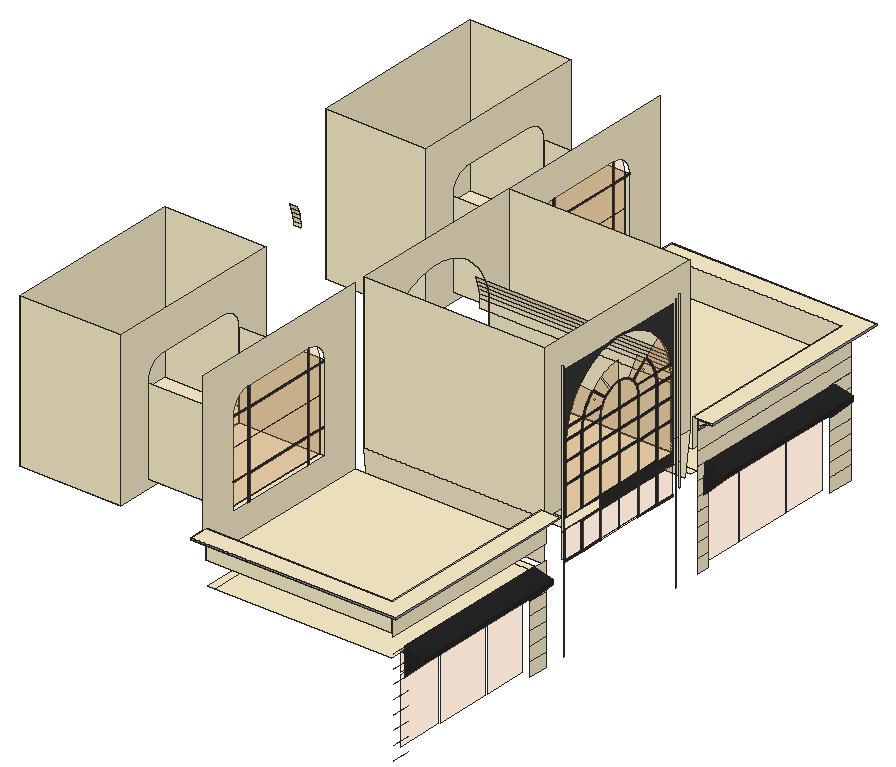
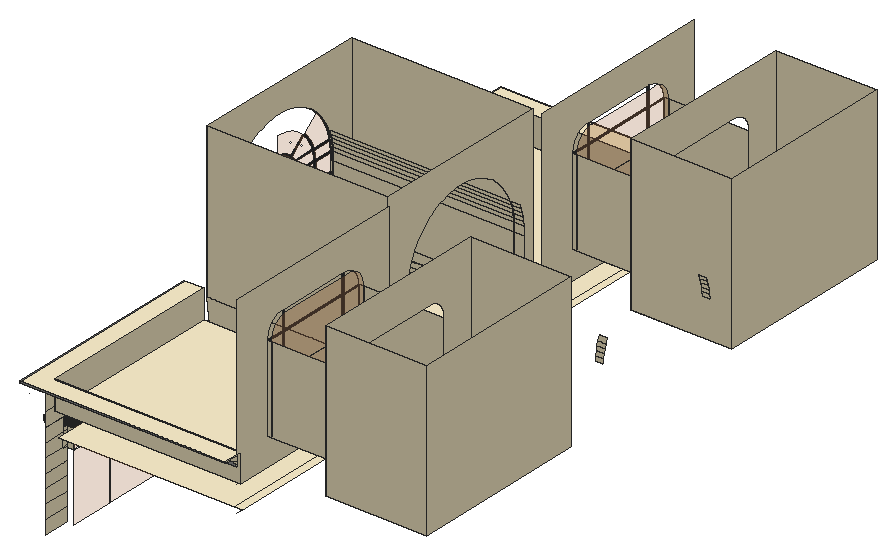
# SketchUp Ruby script. Lengths in inches.
U = 1.inch
M = Sketchup.active_model
def pt(a) = Geom::Point3d.new(a.map { |v| v * U })
def face(e, loops, mat)
  f = e.add_face(loops[0].map { |a| pt(a) })
  loops[1..].each { |l| e.add_face(l.map { |a| pt(a) }).erase! }
  f.material = f.back_material = mat if mat
  f
end
# faces: each face lists its corners as indices into pts; further lists are holes
def faces(e, pts, list, mat = nil) = list.each { |f| face(e, (f[0].is_a?(Array) ? f : [f]).map { |l| l.map { |i| pts[i] } }, mat) }
# xy, xz, yz: faces in a plane at the given z, y or x. An outline is a flat list of corners, or four numbers for a rectangle; further outlines are holes
def ring(l) = l.size == 4 ? [[l[0], l[1]], [l[2], l[1]], [l[2], l[3]], [l[0], l[3]]] : l.each_slice(2).to_a
def flat(e, list, mat, &to3) = list.each { |f| face(e, (f[0].is_a?(Array) ? f : [f]).map { |l| ring(l).map { |u, v| to3.(u, v) } }, mat) }
def xy(e, z, list, mat = nil) = flat(e, list, mat) { |x, y| [x, y, z] }
def xz(e, y, list, mat = nil) = flat(e, list, mat) { |x, z| [x, y, z] }
def yz(e, x, list, mat = nil) = flat(e, list, mat) { |y, z| [x, y, z] }
def lines(e, pts, list) = list.each { |a, b| e.add_line(pt(pts[a]), pt(pts[b])) }
# prism: a flat outline (further loops are holes) pulled along v
def prism(e, loops, v, mat = nil)
  f = face(e, loops, mat); d = Geom::Vector3d.new(v.map { |x| x * U })
  f.pushpull(f.normal.samedirection?(d) ? d.length : -d.length)
end
def box(e, o, s, mat = nil) = prism(e, [[o, [o[0] + s[0], o[1], o[2]], [o[0] + s[0], o[1] + s[1], o[2]], [o[0], o[1] + s[1], o[2]]]], [0, 0, s[2]], mat)
def at(x, y, z, deg = 0) = Geom::Transformation.translation(pt([x, y, z])) * Geom::Transformation.rotation(ORIGIN, Z_AXIS, deg.degrees)
def axes(o, x, y, z) = Geom::Transformation.new([*x, 0, *y, 0, *z, 0, *pt(o).to_a, 1])
def part(name) = M.definitions.add(name)
# library, detail: a bought-in or finely detailed component or shape, given as its bounding box
def library(name, o, s) = part(name).tap { |d| box(d.entities, o, s) }
def detail(e, o, s) = box(e.add_group.entities, o, s)
def put(e, d, t, mat = nil) = e.add_instance(d, t).tap { |i| i.material = mat if mat }
def group(e, t, mat = nil) = e.add_group.tap { |g| g.transformation = t; g.material = mat if mat }.entities
root = M.entities
M.materials.add("Circles_Solid_Black_1K").color = [55, 55, 55]
M.materials.add("D01_Frost_White").color = [255, 242, 206]
M.materials.add("Glass_Safety_01").color = [244, 153, 81]
M.materials["Glass_Safety_01"].alpha = 0.25
M.materials.add("Roofing_02_1K").color = [97, 118, 74]
M.materials.add("ThomThom - Buttons1").color = [48, 49, 53]
M.materials.add("ThomThom - Buttons2").color = [40, 40, 43]
M.materials.add("ThomThom - Hat1").color = [48, 46, 44]
M.materials.add("ThomThom - Hat2").color = [38, 38, 38]
M.materials.add("ThomThom - Waistcoat1").color = [155, 155, 155]
xy(root,42,[[373.34,366.01,374.09,366.03,374.84,366.09,375.59,366.2,376.33,366.35,377.05,366.55,377.77,366.8,378.46,367.09,379.14,367.42,379.79,367.79,380.42,368.21,381.02,368.66,381.59,369.15,382.13,369.68,382.64,370.24,383.1,370.83,383.54,371.44,383.93,372.09,384.28,372.75,384.59,373.44,384.85,374.14,385.07,374.87,385.25,375.6,385.37,376.34,385.45,377.09,385.49,377.84,385.47,378.59,385.41,379.34,385.3,380.09,385.15,380.83,384.95,381.55,384.7,382.27,384.41,382.96,384.08,383.64,383.71,384.29,383.29,384.92,382.84,385.52,382.35,386.09,381.82,386.63,381.26,387.14,380.67,387.6,380.06,388.04,379.41,388.43,378.75,388.78,378.06,389.09,377.36,389.35,376.63,389.57,375.9,389.75,375.16,389.87,374.41,389.95,373.66,389.99,372.91,389.97,372.16,389.91,371.41,389.8,370.67,389.65,369.95,389.45,369.23,389.2,368.54,388.91,367.86,388.58,367.21,388.21,366.58,387.79,365.98,387.34,365.41,386.85,364.87,386.32,364.36,385.76,363.9,385.17,363.46,384.56,363.07,383.91,362.72,383.25,362.41,382.56,362.15,381.86,361.93,381.13,361.75,380.4,361.63,379.66,361.55,378.91,361.51,378.16,361.53,377.41,361.59,376.66,361.7,375.91,361.85,375.17,362.05,374.45,362.3,373.73,362.59,373.04,362.92,372.36,363.29,371.71,363.71,371.08,364.16,370.48,364.65,369.91,365.18,369.37,365.74,368.86,366.33,368.4,366.94,367.96,367.59,367.57,368.25,367.22,368.94,366.91,369.64,366.65,370.37,366.43,371.1,366.25,371.84,366.13,372.59,366.05]],"D01_Frost_White")
xy(root,144,[[252,27,252,258,483,258,483,249,261,249,261,27],[261,27,483,249],[252,498,252,729,261,729,261,507,483,507,483,498],[261,507,483,729],[492,507,516,513],
  [492,705,516,711]],"D01_Frost_White")
xy(root,144,[[483,42,516,234],[483,513,516,705]],"ThomThom - Hat2")
xy(root,174,[[252,24,486,258],[258,294,489,462],[252,498,486,732]],"D01_Frost_White")
xy(root,186,[[258,294,489,462]],"D01_Frost_White")
xy(root,198,[[18,24,144.65,252],[18,504,144.65,732]],"D01_Frost_White")
xy(root,208,[[252,0,252,6,504,6,504,258,510,258,510,0],[252,6,492,18],[492,6,504,258],[492,498,504,738],[504,498,510,738],
  [252,738,504,750],[504,738,510,756],[252,750,504,756]],"D01_Frost_White")
xy(root,210,[[252,0,510,0,510,258,486,258,486,24,252,24],[144.65,66,246,210],[246,66,252,210],[486,498,510,498,510,756,252,756,252,732,486,732],[144.65,546,246,690],
  [246,546,252,690]],"D01_Frost_White")
xz(root,0,[[252,208,510,210]],"ThomThom - Waistcoat1")
xz(root,18,[[252,196,492,202],[252,202,492,208]],"D01_Frost_White")
xz(root,24,[[252,174,486,210],[18,198,144.65,390]],"D01_Frost_White")
xz(root,36,[[492,120,516,144,516,150,492,156]],"ThomThom - Hat2")
xz(root,42,[[492,120,492,144,516,144]],"Roofing_02_1K")
xz(root,66,[[144.65,210,246,318],[246,210,252,318]],"D01_Frost_White")
xz(root,210,[[144.65,210,246,318],[246,210,252,318]],"D01_Frost_White")
xz(root,234,[[492,120,516,144,492,144]],"ThomThom - Hat2")
xz(root,240,[[492,120,492,156,516,150,516,144]],"Roofing_02_1K")
xz(root,252,[[18,198,144.65,390]],"D01_Frost_White")
xz(root,258,[[492,196,498,205,492,202],[492,202,504,208,492,208],[498,205,510,208,504,208]],"D01_Frost_White")
xz(root,264,[[258,198,486,390]],"D01_Frost_White")
xz(root,286,[[490,144,491,174],[490,174,491,362]],"D01_Frost_White")
xz(root,290,[[489,32,490,144],[489,144,490,174],[489,174,490,358]],"D01_Frost_White")
xz(root,294,[[246,174,258,198],[258,186,258,198,486,198,486,264,489,264,489,186],[246,198,258,264],[258,198,486,264],[246,264,258,275.43],
  [258,264,486,275.43],[486,264,489,275.43]],"D01_Frost_White")
xz(root,462,[[258,174,486,186],[486,174,489,186],[258,186,486,264],[486,186,489,264],[246,264,258,275.43],
  [258,264,486,275.43],[486,264,489,275.43]],"D01_Frost_White")
xz(root,466,[[489,32,490,144],[489,144,490,174],[489,174,490,358]],"D01_Frost_White")
xz(root,470,[[490,144,491,174],[490,174,491,362]],"D01_Frost_White")
xz(root,492,[[258,198,486,390]],"D01_Frost_White")
xz(root,498,[[492,196,492,202,498,205],[492,202,492,208,504,208],[498,205,504,208,510,208]],"D01_Frost_White")
xz(root,504,[[18,198,144.65,390]],"D01_Frost_White")
xz(root,507,[[492,120,516,144,492,144],[492,144,516,144,516,150,492,156]],"ThomThom - Hat2")
xz(root,513,[[483,120,492,144]],"D01_Frost_White")
xz(root,513,[[492,120,492,144,516,144]],"ThomThom - Hat2")
xz(root,546,[[144.65,210,246,318],[246,210,252,318]],"D01_Frost_White")
xz(root,690,[[144.65,210,246,318],[246,210,252,318]],"D01_Frost_White")
xz(root,705,[[483,120,492,144]],"D01_Frost_White")
xz(root,705,[[492,120,516,144,492,144]],"ThomThom - Hat2")
xz(root,711,[[492,120,492,144,516,144],[492,144,492,156,516,150,516,144]],"ThomThom - Hat2")
xz(root,732,[[252,174,486,210],[18,198,144.65,390]],"D01_Frost_White")
xz(root,738,[[252,196,492,202],[252,202,492,208]],"D01_Frost_White")
xz(root,756,[[252,208,510,210]],"ThomThom - Waistcoat1")
yz(root,18,[[24,198,252,390],[504,198,732,390]],"D01_Frost_White")
yz(root,144.65,[[[24,198,252,390],[66,210,210,210,210,319.16,209.99,319.52,209.95,320.28,209.89,321.03,209.8,321.79,209.68,322.54,209.54,323.29,209.38,324.03,209.19,324.77,208.98,325.5,208.75,326.22,208.49,326.93,208.21,327.64,207.9,328.33,207.58,329.02,207.23,329.7,206.86,330.36,206.47,331.01,206.05,331.65,205.62,332.27,205.17,332.88,204.69,333.48,204.2,334.06,203.69,334.62,203.16,335.16,202.62,335.69,202.06,336.2,201.48,336.69,200.88,337.17,200.27,337.62,199.65,338.05,199.01,338.47,198.36,338.86,197.7,339.23,197.02,339.58,196.33,339.9,195.64,340.21,194.93,340.49,194.22,340.75,193.5,340.98,192.77,341.19,192.03,341.38,191.29,341.54,190.54,341.68,189.79,341.8,189.03,341.89,188.28,341.95,187.52,341.99,187.16,342,88.1,342,87.71,341.98,86.95,341.93,86.19,341.85,85.4375,341.74,84.68,341.61,83.9375,341.46,83.2,341.28,82.46,341.07,81.73,340.84,81.01,340.59,80.3,340.3125,79.6,340.01,78.91,339.6875,78.23,339.34,77.56,338.97,76.9,338.58,76.26,338.17,75.63,337.74,75.02,337.29,74.42,336.8125,73.84,336.32,73.27,335.81,72.72,335.28,72.19,334.73,71.68,334.16,71.1875,333.58,70.71,332.98,70.26,332.37,69.83,331.74,69.42,331.1,69.03,330.44,68.66,329.77,68.3125,329.09,67.99,328.4,67.6875,327.7,67.41,326.99,67.16,326.27,66.93,325.54,66.72,324.8,66.54,324.0625,66.39,323.32,66.26,322.5625,66.15,321.81,66.07,321.05,66.02,320.29,66,319.9]],[[504,198,732,390],[546,210,690,210,690,319.87,689.98,320.29,689.93,321.05,689.85,321.81,689.74,322.5625,689.61,323.31,689.45,324.0625,689.27,324.8,689.07,325.54,688.84,326.27,688.58,326.98,688.31,327.7,688.01,328.4,687.68,329.09,687.34,329.77,686.97,330.4375,686.58,331.09,686.17,331.73,685.73,332.36,685.28,332.98,684.81,333.57,684.3125,334.16,683.8,334.72,683.27,335.27,682.72,335.8,682.16,336.3125,681.57,336.81,680.98,337.28,680.36,337.73,679.73,338.17,679.09,338.58,678.4375,338.97,677.77,339.34,677.09,339.68,676.4,340.01,675.7,340.31,674.98,340.58,674.27,340.84,673.54,341.07,672.8,341.27,672.0625,341.45,671.31,341.61,670.5625,341.74,669.81,341.85,669.05,341.93,668.29,341.98,667.87,342,567.32,342,566.93,341.98,566.17,341.91,565.41,341.8125,564.65,341.6875,563.9,341.54,563.15,341.37,562.41,341.17,561.68,340.95,560.95,340.7,560.23,340.43,559.53,340.13,558.83,339.8125,558.14,339.47,557.47,339.1,556.81,338.71,556.16,338.3,555.53,337.87,554.91,337.42,554.31,336.94,553.72,336.45,553.15,335.93,552.6,335.4,552.07,334.85,551.55,334.28,551.06,333.69,550.58,333.09,550.13,332.47,549.7,331.84,549.29,331.19,548.9,330.53,548.53,329.86,548.1875,329.17,547.87,328.47,547.57,327.77,547.3,327.05,547.05,326.32,546.83,325.59,546.63,324.85,546.46,324.1,546.3125,323.35,546.1875,322.59,546.09,321.83,546.02,321.07,546,320.68]]],"D01_Frost_White")
yz(root,246,[[66,210,210,275.23],[546,210,690,275.23],[66,275.23,66,319.9,66.02,320.29,66.07,321.05,66.15,321.81,66.26,322.5625,66.39,323.32,66.54,324.0625,66.72,324.8,66.93,325.54,67.16,326.27,67.41,326.99,67.6875,327.7,67.99,328.4,68.3125,329.09,68.66,329.77,69.03,330.44,69.42,331.1,69.83,331.74,70.26,332.37,70.71,332.98,71.1875,333.58,71.68,334.16,72.19,334.73,72.72,335.28,73.27,335.81,73.84,336.32,74.42,336.8125,75.02,337.29,75.63,337.74,76.26,338.17,76.9,338.58,77.56,338.97,78.23,339.34,78.91,339.6875,79.6,340.01,80.3,340.3125,81.01,340.59,81.73,340.84,82.46,341.07,83.2,341.28,83.9375,341.46,84.68,341.61,85.4375,341.74,86.19,341.85,86.95,341.93,87.71,341.98,88.1,342,187.16,342,187.52,341.99,188.28,341.95,189.03,341.89,189.79,341.8,190.54,341.68,191.29,341.54,192.03,341.38,192.77,341.19,193.5,340.98,194.22,340.75,194.93,340.49,195.64,340.21,196.33,339.9,197.02,339.58,197.7,339.23,198.36,338.86,199.01,338.47,199.65,338.05,200.27,337.62,200.88,337.17,201.48,336.69,202.06,336.2,202.62,335.69,203.16,335.16,203.69,334.62,204.2,334.06,204.69,333.48,205.17,332.88,205.62,332.27,206.05,331.65,206.47,331.01,206.86,330.36,207.23,329.7,207.58,329.02,207.9,328.33,208.21,327.64,208.49,326.93,208.75,326.22,208.98,325.5,209.19,324.77,209.38,324.03,209.54,323.29,209.68,322.54,209.8,321.79,209.89,321.03,209.95,320.28,209.99,319.52,210,319.16,210,275.23],[546,275.23,546,320.68,546.02,321.07,546.09,321.83,546.1875,322.59,546.3125,323.35,546.46,324.1,546.63,324.85,546.83,325.59,547.05,326.32,547.3,327.05,547.57,327.77,547.87,328.47,548.1875,329.17,548.53,329.86,548.9,330.53,549.29,331.19,549.7,331.84,550.13,332.47,550.58,333.09,551.06,333.69,551.55,334.28,552.07,334.85,552.6,335.4,553.15,335.93,553.72,336.45,554.31,336.94,554.91,337.42,555.53,337.87,556.16,338.3,556.81,338.71,557.47,339.1,558.14,339.47,558.83,339.8125,559.53,340.13,560.23,340.43,560.95,340.7,561.68,340.95,562.41,341.17,563.15,341.37,563.9,341.54,564.65,341.6875,565.41,341.8125,566.17,341.91,566.93,341.98,567.32,342,667.87,342,668.29,341.98,669.05,341.93,669.81,341.85,670.5625,341.74,671.31,341.61,672.0625,341.45,672.8,341.27,673.54,341.07,674.27,340.84,674.98,340.58,675.7,340.31,676.4,340.01,677.09,339.68,677.77,339.34,678.4375,338.97,679.09,338.58,679.73,338.17,680.36,337.73,680.98,337.28,681.57,336.81,682.16,336.3125,682.72,335.8,683.27,335.27,683.8,334.72,684.3125,334.16,684.81,333.57,685.28,332.98,685.73,332.36,686.17,331.73,686.58,331.09,686.97,330.4375,687.34,329.77,687.68,329.09,688.01,328.4,688.31,327.7,688.58,326.98,688.84,326.27,689.07,325.54,689.27,324.8,689.45,324.0625,689.61,323.31,689.74,322.5625,689.85,321.81,689.93,321.05,689.98,320.29,690,319.87,690,275.23]],"Glass_Safety_01")
yz(root,252,[[[24,174,258,174,258,384,18,384,18,210,24,210],[66,210,66,318,65.98,318.76,65.98,319.53,66,319.9,66.02,320.29,66.07,321.05,66.15,321.81,66.26,322.5625,66.39,323.32,66.54,324.0625,66.72,324.8,66.93,325.54,67.16,326.27,67.41,326.99,67.6875,327.7,67.99,328.4,68.3125,329.09,68.66,329.77,69.03,330.44,69.42,331.1,69.83,331.74,70.26,332.37,70.71,332.98,71.1875,333.58,71.68,334.16,72.19,334.73,72.72,335.28,73.27,335.81,73.84,336.32,74.42,336.8125,75.02,337.29,75.63,337.74,76.26,338.17,76.9,338.58,77.56,338.97,78.23,339.34,78.91,339.6875,79.6,340.01,80.3,340.3125,81.01,340.59,81.73,340.84,82.46,341.07,83.2,341.28,83.9375,341.46,84.68,341.61,85.4375,341.74,86.19,341.85,86.95,341.93,87.71,341.98,88.1,342,88.47,342.02,89.24,342.02,90,342,186,342,186.76,342.01,187.16,342,187.52,341.99,188.28,341.95,189.03,341.89,189.79,341.8,190.54,341.68,191.29,341.54,192.03,341.38,192.77,341.19,193.5,340.98,194.22,340.75,194.93,340.49,195.64,340.21,196.33,339.9,197.02,339.58,197.7,339.23,198.36,338.86,199.01,338.47,199.65,338.05,200.27,337.62,200.88,337.17,201.48,336.69,202.06,336.2,202.62,335.69,203.16,335.16,203.69,334.62,204.2,334.06,204.69,333.48,205.17,332.88,205.62,332.27,206.05,331.65,206.47,331.01,206.86,330.36,207.23,329.7,207.58,329.02,207.9,328.33,208.21,327.64,208.49,326.93,208.75,326.22,208.98,325.5,209.19,324.77,209.38,324.03,209.54,323.29,209.68,322.54,209.8,321.79,209.89,321.03,209.95,320.28,209.99,319.52,210,319.16,210.01,318.76,210,318,210,210]],[[498,174,732,174,732,210,738,210,738,384,498,384],[546,210,546,318,545.97,318.77,545.96,319.53,545.98,320.3,546,320.68,546.02,321.07,546.09,321.83,546.1875,322.59,546.3125,323.35,546.46,324.1,546.63,324.85,546.83,325.59,547.05,326.32,547.3,327.05,547.57,327.77,547.87,328.47,548.1875,329.17,548.53,329.86,548.9,330.53,549.29,331.19,549.7,331.84,550.13,332.47,550.58,333.09,551.06,333.69,551.55,334.28,552.07,334.85,552.6,335.4,553.15,335.93,553.72,336.45,554.31,336.94,554.91,337.42,555.53,337.87,556.16,338.3,556.81,338.71,557.47,339.1,558.14,339.47,558.83,339.8125,559.53,340.13,560.23,340.43,560.95,340.7,561.68,340.95,562.41,341.17,563.15,341.37,563.9,341.54,564.65,341.6875,565.41,341.8125,566.17,341.91,566.93,341.98,567.32,342,567.7,342.02,568.47,342.04,569.23,342.03,570,342,666,342,666.76,342.02,667.53,342.01,667.87,342,668.29,341.98,669.05,341.93,669.81,341.85,670.5625,341.74,671.31,341.61,672.0625,341.45,672.8,341.27,673.54,341.07,674.27,340.84,674.98,340.58,675.7,340.31,676.4,340.01,677.09,339.68,677.77,339.34,678.4375,338.97,679.09,338.58,679.73,338.17,680.36,337.73,680.98,337.28,681.57,336.81,682.16,336.3125,682.72,335.8,683.27,335.27,683.8,334.72,684.3125,334.16,684.81,333.57,685.28,332.98,685.73,332.36,686.17,331.73,686.58,331.09,686.97,330.4375,687.34,329.77,687.68,329.09,688.01,328.4,688.31,327.7,688.58,326.98,688.84,326.27,689.07,325.54,689.27,324.8,689.45,324.0625,689.61,323.31,689.74,322.5625,689.85,321.81,689.93,321.05,689.98,320.29,690,319.87,690.01,319.53,690.02,318.76,690,318,690,210]],[18,196,12,205,18,202],[738,196,738,202,744,205],[18,202,6,208,18,208],
  [738,202,738,208,750,208],[12,205,0,208,6,208],[744,205,750,208,756,208],[0,208,18,210],[738,208,756,210]],"D01_Frost_White")
yz(root,252,[[[90,210,92,210,92,242,184,242,184,210,186,210,186,242,210,242,210,244,186,244,186,316,210,316,210,318,186,318,186,342,184,342,184,318,92,318,92,342,90,342,90,318,66,318,66,316,90,316,90,244,66,244,66,242,90,242],[92,244,184,316]],[[570,210,572,210,572,242,664,242,664,210,666,210,666,242,690,242,690,244,666,244,666,316,690,316,690,318,666,318,666,342,664,342,664,318,572,318,572,342,570,342,570,318,546,318,546,316,570,316,570,244,546,244,546,242,570,242],[572,244,664,316]]],"ThomThom - Buttons1")
yz(root,258,[[294,174,462,186],[264,198,294,198,294,275.43,294.49,280.53,295.37,285.98,296.61,291.37,298.2,296.65,300.13,301.83,302.4,306.86,304.99,311.74,307.89,316.43,311.1,320.93,314.59,325.2,318.36,329.24,322.39,333.02,326.65,336.53,331.13,339.75,335.82,342.67,340.6875,345.28,345.71,347.5625,350.88,349.51,356.16,351.12,361.54,352.375,366.99,353.28,372.48,353.82,378,354,383.52,353.82,389.01,353.28,394.46,352.375,399.84,351.12,405.12,349.51,410.29,347.5625,415.3125,345.28,420.18,342.67,424.87,339.75,429.35,336.53,433.61,333.02,437.64,329.24,441.41,325.2,444.9,320.93,448.11,316.43,451.01,311.74,453.6,306.86,455.87,301.83,457.8,296.65,459.39,291.37,460.63,285.98,461.51,280.53,462,275.43,462,198,492,198,492,390,264,390]],"D01_Frost_White")
yz(root,483,[[513,34,573,118],[575,34,647,118],[649,34,705,118],[42,36,102,118],[104,36,176,118],
  [178,36,234,118],[42,120,102,144],[104,120,176,144],[178,120,234,144],[513,120,573,144],
  [575,120,647,144],[649,120,705,144]],"Glass_Safety_01")
yz(root,486,[[24,174,258,210],[498,174,732,210],[264,198,264,390,492,390,492,198,462,198,462,275.43,461.51,280.53,460.63,285.98,459.39,291.37,457.8,296.65,455.87,301.83,453.6,306.86,451.01,311.74,448.11,316.43,444.9,320.93,441.41,325.2,437.64,329.24,433.61,333.02,429.35,336.53,424.87,339.75,420.18,342.67,415.3125,345.28,410.29,347.5625,405.12,349.51,399.84,351.12,394.46,352.375,389.01,353.28,383.52,353.82,378,354,372.48,353.82,366.99,353.28,361.54,352.375,356.16,351.12,350.88,349.51,345.71,347.5625,340.6875,345.28,335.82,342.67,331.13,339.75,326.65,336.53,322.39,333.02,318.36,329.24,314.59,325.2,311.1,320.93,307.89,316.43,304.99,311.74,302.4,306.86,300.13,301.83,298.2,296.65,296.61,291.37,295.37,285.98,294.49,280.53,294,275.43,294,198]],"D01_Frost_White")
yz(root,489,[[294,275.43,294.49,280.53,295.37,285.98,295.42,286.1875,295.88,288.1875,296.61,291.37,298.2,296.65,300.13,301.83,302.4,306.86,304.99,311.74,307.89,316.43,311.1,320.93,314.59,325.2,316.37,327.1,317.4,328.21,318.36,329.24,322.39,333.02,326.65,336.53,331.13,339.75,333.04,340.94,334.65,341.94,335.82,342.67,340.6875,345.28,345.71,347.5625,350.88,349.51,356.16,351.12,361.54,352.375,366.99,353.28,372.48,353.82,377,353.97,377,354,294,354],[462,275.43,462,354,379,354,379,353.97,383.52,353.82,389.01,353.28,394.46,352.375,399.84,351.12,405.12,349.51,410.29,347.5625,415.3125,345.28,420.18,342.67,421.22,342.02,422.83,341.02,424.87,339.75,429.35,336.53,433.61,333.02,437.64,329.24,438.53,328.29,439.55,327.19,441.41,325.2,444.9,320.93,448.11,316.43,451.01,311.74,453.6,306.86,455.87,301.83,457.8,296.65,459.39,291.37,460.12,288.1875,460.58,286.1875,460.63,285.98,461.51,280.53]],"Circles_Solid_Black_1K")
yz(root,489,[[294,264,294,275.43,293.96,275.04,293.8,269.52],[462,264,462.2,269.52,462.0625,274.1875,462,274.1875],[462,274.1875,462.0625,274.1875,462.04,275.04,462,275.43]],"D01_Frost_White")
yz(root,489,[[348.5,136.9,377,138.9],[377,136.9,379,138.9],[379,136.9,407.5,138.9],[294,138.9,318,174],[320,138.9,347.5,172],
  [348.5,138.9,377,172],[377,138.9,379,172],[379,138.9,407.5,172],[408.5,138.9,436,172],[438,138.9,462,174],
  [294,186,318,222.1875],[438,186,462,222.1875],[320,188,347.5,222.1875],[348.5,188,377,222.1875],[379,188,407.5,222.1875],
  [408.5,188,436,222.1875],[294,224.1875,318,248.1875],[320,224.1875,347.5,248.1875],[348.5,224.1875,377,248.1875],[379,224.1875,407.5,248.1875],
  [408.5,224.1875,436,248.1875],[438,224.1875,462,248.1875],[294,250.1875,318,272.1875],[320,250.1875,347.5,272.1875],[348.5,250.1875,377,272.1875],
  [379,250.1875,407.5,272.1875],[408.5,250.1875,436,272.1875],[438,250.1875,462,272.1875],[294,274.1875,318,274.1875,318,274.28,318.3,277.47,318.94,281.37,319.82,285.22,320.11,286.1875,295.42,286.1875,295.37,285.98,294.49,280.53,294,275.43],[320,274.1875,347.5,274.1875,347.56,276.1,347.74,278.01,348.04,279.9,348.46,281.77,348.99,283.61,349.64,285.42,349.98,286.1875,322.2,286.1875,321.75,284.7,320.9,280.98,320.29,277.22],
  [[348.5,274.1875,377,274.1875,377,303.66,376.15,303.63,374.3,303.46,372.47,303.17,370.66,302.76,368.88,302.24,367.14,301.62,365.44,300.88,363.79,300.04,362.19,299.1,360.66,298.05,359.2,296.92,357.81,295.69,356.5,294.38,355.27,292.99,354.13,291.53,353.09,290,352.15,288.4,352.04,288.1875,351.31,286.75,351.07,286.1875,350.57,285.05,349.94,283.3,349.43,281.52,349.02,279.72,348.73,277.89,348.56,276.04],[347.5,188,348.5,222.1875],[347.5,224.1875,348.5,248.1875],[347.5,250.1875,348.5,272.1875]],[379,274.1875,407.5,274.1875,407.44,276.04,407.27,277.89,406.98,279.72,406.57,281.52,406.06,283.3,405.43,285.05,404.93,286.1875,404.69,286.75,403.96,288.1875,403.85,288.4,402.91,290,401.87,291.53,400.73,292.99,399.5,294.38,398.19,295.69,396.8,296.92,395.34,298.05,393.81,299.1,392.21,300.04,390.56,300.88,388.86,301.62,387.12,302.24,385.34,302.76,383.53,303.17,381.7,303.46,379.85,303.63,379,303.66],[408.5,274.1875,436,274.1875,435.71,277.22,435.1,280.98,434.25,284.7,433.8,286.1875,406.02,286.1875,406.36,285.42,407.01,283.61,407.54,281.77,407.96,279.9,408.26,278.01,408.44,276.1],[438,274.1875,462,274.1875,462,275.43,461.51,280.53,460.63,285.98,460.58,286.1875,435.89,286.1875,436.18,285.22,437.06,281.37,437.7,277.47,438,274.28],[295.88,288.1875,320.71,288.1875,320.96,289,322.34,292.69,323.96,296.29,325.81,299.78,327.89,303.13,330.18,306.35,332.68,309.4,334.82,311.7,316.37,327.1,314.59,325.2,311.1,320.93,307.89,316.43,304.99,311.74,302.4,306.86,300.13,301.83,298.2,296.65,296.61,291.37],
  [[322.8,288.1875,350.92,288.1875,351.27,288.88,352.25,290.53,353.32,292.12,354.5,293.63,355.77,295.07,357.12,296.42,358.56,297.6875,360.07,298.86,361.66,299.94,363.31,300.92,365.01,301.79,366.77,302.55,368.57,303.2,370.41,303.73,372.28,304.15,374.18,304.45,376.08,304.63,377,304.66,377,327.95,374.1875,327.86,370.39,327.49,366.625,326.86,362.91,325.99,359.26,324.89,355.6875,323.54,352.21,321.96,350.4,320.99,364.82,301.79,363.12,300.92,348.72,320.08,345.61,318.14,342.51,315.91,339.57,313.49,337.43,311.47,356.25,295.74,355.58,295.07,355.22,294.67,336.36,310.42,334.18,308.09,331.77,305.13,329.55,302.03,327.54,298.78,325.75,295.41,324.1875,291.93,322.85,288.36],[338.87,299.58,338.92,299.66,338.96,299.71]],[[405.08,288.1875,433.2,288.1875,433.15,288.36,431.8125,291.93,430.25,295.41,428.46,298.78,426.45,302.03,424.23,305.13,421.82,308.09,419.56,310.51,400.58,294.67,401.5,293.63,402.68,292.12,403.75,290.53,404.73,288.88],[417.13,299.58,417.04,299.71,417.08,299.66]],[435.29,288.1875,460.12,288.1875,459.39,291.37,457.8,296.65,455.87,301.83,453.6,306.86,451.01,311.74,448.11,316.43,444.9,320.93,441.41,325.2,439.55,327.19,421.1,311.79,423.32,309.4,425.82,306.35,428.11,303.13,430.19,299.78,432.04,296.29,433.66,292.69,435.04,289],[399.56,295.74,418.48,311.56,416.43,313.49,413.49,315.91,410.39,318.14,407.15,320.16,392.69,300.92,394.34,299.94,395.93,298.86,397.44,297.6875,398.88,296.42]],"Glass_Safety_01")
yz(root,489,[[294,136.9,318,138.9],[320,136.9,347.5,138.9],[408.5,136.9,436,138.9],[438,136.9,462,138.9],[355.22,294.67,355.58,295.07,356.25,295.74,337.43,311.47,336.79,310.875,336.36,310.42],
  [400.58,294.67,419.56,310.51,418.48,311.56,399.56,295.74,400.23,295.07]],"ThomThom - Buttons1")
yz(root,489,[[318,136.9,320,138.9],[347.5,136.9,348.5,138.9],[407.5,136.9,408.5,138.9],[436,136.9,438,138.9],[318,138.9,320,138.9,320,172,347.5,172,347.5,174,318,174],
  [347.5,138.9,348.5,172],[407.5,138.9,408.5,172],[436,138.9,438,138.9,438,174,408.5,174,408.5,172,436,172],[347.5,172,348.5,174],[348.5,172,377,174],
  [377,172,379,174],[379,172,407.5,174],[407.5,172,408.5,174],[318,186,347.5,186,347.5,188,320,188,320,222.1875,347.5,222.1875,347.5,224.1875,320,224.1875,320,248.1875,347.5,248.1875,347.5,250.1875,320,250.1875,320,272.1875,347.5,272.1875,347.5,274.1875,320,274.1875,320.29,277.22,320.9,280.98,321.75,284.7,322.2,286.1875,349.98,286.1875,350.4,287.17,350.92,288.1875,322.8,288.1875,322.85,288.36,324.1875,291.93,325.75,295.41,327.54,298.78,329.55,302.03,331.77,305.13,334.18,308.09,336.36,310.42,336.25,310.51,334.82,311.7,332.68,309.4,330.18,306.35,327.89,303.13,325.81,299.78,323.96,296.29,322.34,292.69,320.96,289,320.71,288.1875,295.88,288.1875,295.42,286.1875,320.11,286.1875,319.82,285.22,318.94,281.37,318.3,277.47,318,274.28,318,274.1875,294,274.1875,294,272.1875,318,272.1875,318,250.1875,294,250.1875,294,248.1875,318,248.1875,318,224.1875,294,224.1875,294,222.1875,318,222.1875],[347.5,186,348.5,188],
  [348.5,186,377,188],[377,186,379,188],[379,186,407.5,188],[408.5,186,438,186,438,222.1875,462,222.1875,462,224.1875,438,224.1875,438,248.1875,462,248.1875,462,250.1875,438,250.1875,438,272.1875,462,272.1875,462,274.1875,438,274.1875,438,274.28,437.7,277.47,437.06,281.37,436.18,285.22,435.89,286.1875,460.58,286.1875,460.12,288.1875,435.29,288.1875,435.04,289,433.66,292.69,432.04,296.29,430.19,299.78,428.11,303.13,425.82,306.35,423.32,309.4,421.1,311.79,419.56,310.51,421.82,308.09,424.23,305.13,426.45,302.03,428.46,298.78,430.25,295.41,431.8125,291.93,433.15,288.36,433.2,288.1875,405.08,288.1875,405.6,287.17,406.02,286.1875,433.8,286.1875,434.25,284.7,435.1,280.98,435.71,277.22,436,274.1875,408.5,274.1875,408.5,272.1875,436,272.1875,436,250.1875,408.5,250.1875,408.5,248.1875,436,248.1875,436,224.1875,408.5,224.1875,408.5,222.1875,436,222.1875,436,188,408.5,188],[407.5,186,408.5,188],
  [347.5,188,348.5,222.1875],[377,188,379,188,379,222.1875,407.5,222.1875,407.5,224.1875,379,224.1875,379,248.1875,407.5,248.1875,407.5,250.1875,379,250.1875,379,272.1875,407.5,272.1875,407.5,274.1875,379,274.1875,379,303.66,378,303.6875,377,303.66,377,274.1875,348.5,274.1875,348.5,272.1875,377,272.1875,377,250.1875,348.5,250.1875,348.5,248.1875,377,248.1875,377,224.1875,348.5,224.1875,348.5,222.1875,377,222.1875],[407.5,188,408.5,222.1875],[347.5,222.1875,348.5,224.1875],[407.5,222.1875,408.5,224.1875],
  [347.5,224.1875,348.5,248.1875],[407.5,224.1875,408.5,248.1875],[347.5,248.1875,348.5,250.1875],[407.5,248.1875,408.5,250.1875],[347.5,250.1875,348.5,272.1875],
  [407.5,250.1875,408.5,272.1875],[347.5,272.1875,348.5,274.1875],[407.5,272.1875,408.5,274.1875],[347.5,274.1875,348.5,274.1875,348.56,276.04,348.73,277.89,349.02,279.72,349.43,281.52,349.94,283.3,350.57,285.05,351.07,286.1875,349.98,286.1875,349.64,285.42,348.99,283.61,348.46,281.77,348.04,279.9,347.74,278.01,347.56,276.1],[407.5,274.1875,408.5,274.1875,408.44,276.1,408.26,278.01,407.96,279.9,407.54,281.77,407.01,283.61,406.36,285.42,406.02,286.1875,404.93,286.1875,405.43,285.05,406.06,283.3,406.57,281.52,406.98,279.72,407.27,277.89,407.44,276.04],
  [349.98,286.1875,351.07,286.1875,351.31,286.75,352.04,288.1875,350.92,288.1875,350.4,287.17],[404.93,286.1875,406.02,286.1875,405.6,287.17,405.08,288.1875,403.96,288.1875,404.69,286.75],[350.92,288.1875,352.04,288.1875,352.15,288.4,353.09,290,354.13,291.53,355.27,292.99,356.5,294.38,357.81,295.69,359.2,296.92,360.66,298.05,362.19,299.1,363.79,300.04,365.44,300.88,367.14,301.62,368.88,302.24,370.66,302.76,372.47,303.17,374.3,303.46,376.15,303.63,377,303.66,377,304.66,376.08,304.63,374.18,304.45,372.28,304.15,370.41,303.73,368.57,303.2,366.77,302.55,365.01,301.79,363.31,300.92,361.66,299.94,360.07,298.86,358.56,297.6875,357.12,296.42,355.77,295.07,354.5,293.63,353.32,292.12,352.25,290.53,351.27,288.88],[403.96,288.1875,405.08,288.1875,404.73,288.88,403.75,290.53,402.68,292.12,401.5,293.63,400.58,294.67,399.56,295.74,398.88,296.42,397.44,297.6875,395.93,298.86,394.34,299.94,392.69,300.92,390.99,301.79,389.23,302.55,387.43,303.2,385.59,303.73,383.72,304.15,381.82,304.45,379.92,304.63,379,304.66,379,303.66,379.85,303.63,381.7,303.46,383.53,303.17,385.34,302.76,387.12,302.24,388.86,301.62,390.56,300.88,392.21,300.04,393.81,299.1,395.34,298.05,396.8,296.92,398.19,295.69,399.5,294.38,400.73,292.99,401.87,291.53,402.91,290,403.85,288.4],[400.58,294.67,400.23,295.07,399.56,295.74]],"ThomThom - Buttons2")
yz(root,489,[[347.5,174,348.5,186],[348.5,174,377,186],[377,174,379,186],[379,174,407.5,186],[407.5,174,408.5,186],
  [408.5,174,462,186]],"ThomThom - Hat1")
yz(root,492,[[234,34.38,258,51.57],[498,34.8,513,52.2],[705,34.8,738,52.2],[234,51.57,258,68.76],[498,52.2,513,69.6],
  [705,52.2,738,69.6],[234,68.76,258,85.95],[498,69.6,513,87],[705,69.6,738,87],[234,85.95,258,103.14],
  [498,87,513,104.4],[705,87,738,104.4],[234,103.14,258,103.14,258,120.32,240,120.32,240,120,234,120],[498,104.4,513,104.4,513,120,507,120,507,121.8,498,121.8],[705,104.4,738,104.4,738,121.8,711,121.8,711,120,705,120],
  [36,120,42,144],[234,120,240,120.32],[507,120,513,121.8],[705,120,711,121.8],[234,120.32,240,137.51],
  [240,120.32,258,137.51],[498,121.8,507,139.2],[507,121.8,513,139.2],[705,121.8,711,139.2],[711,121.8,738,139.2],
  [234,137.51,240,144],[240,137.51,258,154.7],[498,139.2,507,139.2,507,156,711,156,711,139.2,738,139.2,738,174,498,174],[507,139.2,513,144],[705,139.2,711,144],
  [18,174,258,196],[498,174,738,196],[18,196,258,202],[498,196,738,202],[18,202,258,208],
  [498,202,738,208]],"D01_Frost_White")
yz(root,510,[[0,208,258,210],[498,208,756,210]],"ThomThom - Waistcoat1")
yz(root,516,[[36,144,240,150],[507,144,711,150]],"ThomThom - Hat2")
p = [[492,42,120],[516,42,144],[516,36,144],[492,36,120],[516,234,144],[492,234,120],
  [492,240,120],[516,240,144],[492,513,120],[516,513,144],[516,507,144],[492,507,120],
  [492,711,120],[516,711,144],[516,705,144],[492,705,120],[261,267,144],[258,264,198],
  [486,264,198],[483,267,144],[483,489,144],[486,492,198],[258,492,198],[261,489,144],
  [492,36,156],[516,36,150],[516,240,150],[492,240,156],[516,711,150],[492,711,156],
  [492,507,156],[516,507,150],[252,12,205],[252,18,196],[492,18,196],[498,12,205],
  [492,258,196],[498,258,205],[492,18,202],[492,738,196],[498,744,205],[498,498,205],
  [492,498,196],[252,738,196],[252,744,205],[492,738,202],[252,18,202],[492,258,202],
  [492,498,202],[252,738,202],[252,0,208],[510,0,208],[510,258,208],[252,6,208],
  [504,6,208],[492,6,208],[504,258,208],[504,498,208],[504,750,208],[504,738,208],
  [510,498,208],[510,756,208],[510,738,208],[252,750,208],[252,756,208],[504,756,208],
  [21,294.49,280.53],[21,294,275.43],[12,294,275.43],[12,294.49,280.53],[258,294.49,280.53],[258,294,275.43],
  [246,294,275.43],[246,294.49,280.53],[486,294.49,280.53],[486,294,275.43],[489,294.49,280.53],[489,294,275.43],
  [21,462,275.43],[21,461.51,280.53],[12,461.51,280.53],[12,462,275.43],[258,462,275.43],[258,461.51,280.53],
  [246,461.51,280.53],[246,462,275.43],[486,462,275.43],[486,461.51,280.53],[489,462,275.43],[489,461.51,280.53],
  [21,295.37,285.98],[12,295.37,285.98],[258,295.37,285.98],[246,295.37,285.98],[486,295.37,285.98],[489,295.37,285.98],
  [21,460.63,285.98],[12,460.63,285.98],[258,460.63,285.98],[246,460.63,285.98],[486,460.63,285.98],[489,460.63,285.98],
  [21,296.61,291.37],[12,296.61,291.37],[258,296.61,291.37],[246,296.61,291.37],[486,296.61,291.37],[489,295.42,286.1875],
  [489,296.61,291.37],[489,295.88,288.1875],[21,459.39,291.37],[12,459.39,291.37],[258,459.39,291.37],[246,459.39,291.37],
  [486,459.39,291.37],[489,460.12,288.1875],[489,459.39,291.37],[489,460.58,286.1875],[21,298.2,296.65],[12,298.2,296.65],
  [258,298.2,296.65],[246,298.2,296.65],[486,298.2,296.65],[489,298.2,296.65],[21,457.8,296.65],[12,457.8,296.65],
  [258,457.8,296.65],[246,457.8,296.65],[486,457.8,296.65],[489,457.8,296.65],[21,300.13,301.83],[12,300.13,301.83],
  [258,300.13,301.83],[246,300.13,301.83],[486,300.13,301.83],[489,300.13,301.83],[21,455.87,301.83],[12,455.87,301.83],
  [258,455.87,301.83],[246,455.87,301.83],[486,455.87,301.83],[489,455.87,301.83],[252,738.1,176.27],[252,738,176.27],
  [492,18,34.51],[492,42,34.51],[492,18,51.77],[492,42,51.77],[492,18,69.03],[492,42,69.03],
  [492,18,86.29],[492,42,86.29],[492,18,103.54],[492,42,103.54],[492,18,120.8],[492,42,120.8],
  [492,18,138.06],[492,42,138.06],[492,18,155.32],[492,42,155.32],[492,178,144],[492,176,144],
  [492,104,144],[492,102,144],[489,463.28,274.1875],[489,462.0625,274.1875],[504,750,196],[504.07,750,196],
  [489,294,174],[491,462,174],[489,295.37,286.1875],[489,460.37,288.1875],[489,295.42,288.1875],[252,729,144],
  [252,738,144],[492,234,154.7],[492,240,154.7],[492,738,156.6],[492,705,156.6],[492,513,156.6],
  [492,498,156.6]]
faces(root,p,[[0,1,2,3],[4,5,6,7],[8,9,10,11],[12,13,14,15],[24,25,26,27],[28,29,30,31]],"ThomThom - Hat2")
faces(root,p,[[16,17,18,19],[20,21,22,23],[34,35,38],[40,39,45],[38,35,32,46],[47,37,35,38],[45,40,41,48],[49,44,40,45],
  [53,32,35,54,55],[54,35,37,56],[57,41,40,58,59],[58,40,44,63],[66,67,68,69],[70,71,72,73],[74,75,71,70],[76,77,75,74],
  [78,79,80,81],[82,83,84,85],[86,87,83,82],[88,89,87,86],[90,66,69,91],[92,70,73,93],[94,74,70,92],[95,76,74,94],
  [79,96,97,80],[83,98,99,84],[87,100,98,83],[89,101,100,87],[102,90,91,103],[104,92,93,105],[106,94,92,104],[107,95,94,106,108,109],
  [96,110,111,97],[98,112,113,99],[100,114,112,98],[115,116,114,100,101,117],[118,102,103,119],[120,104,105,121],[122,106,104,120],[123,108,106,122],
  [110,124,125,111],[112,126,127,113],[114,128,126,112],[116,129,128,114],[130,118,119,131],[132,120,121,133],[134,122,120,132],[135,123,122,134],
  [124,136,137,125],[126,138,139,127],[128,140,138,126],[129,141,140,128]],"D01_Frost_White")
faces(root,p,[[32,33,34,35],[36,37,35,34],[39,40,41,42],[43,44,40,39],[50,32,35,51],[37,52,51,35],[60,41,40,61,62],[44,64,65,61,40]],"ThomThom - Waistcoat1")
lines(root,p,[[142,143],[144,145],[146,147],[148,149],[150,151],[152,153],[154,155],[156,157],[158,159],[160,161],[162,163],[164,165],
  [166,167],[168,169],[107,170],[115,171],[109,172],[173,174],[175,176],[177,178],[179,180]])
